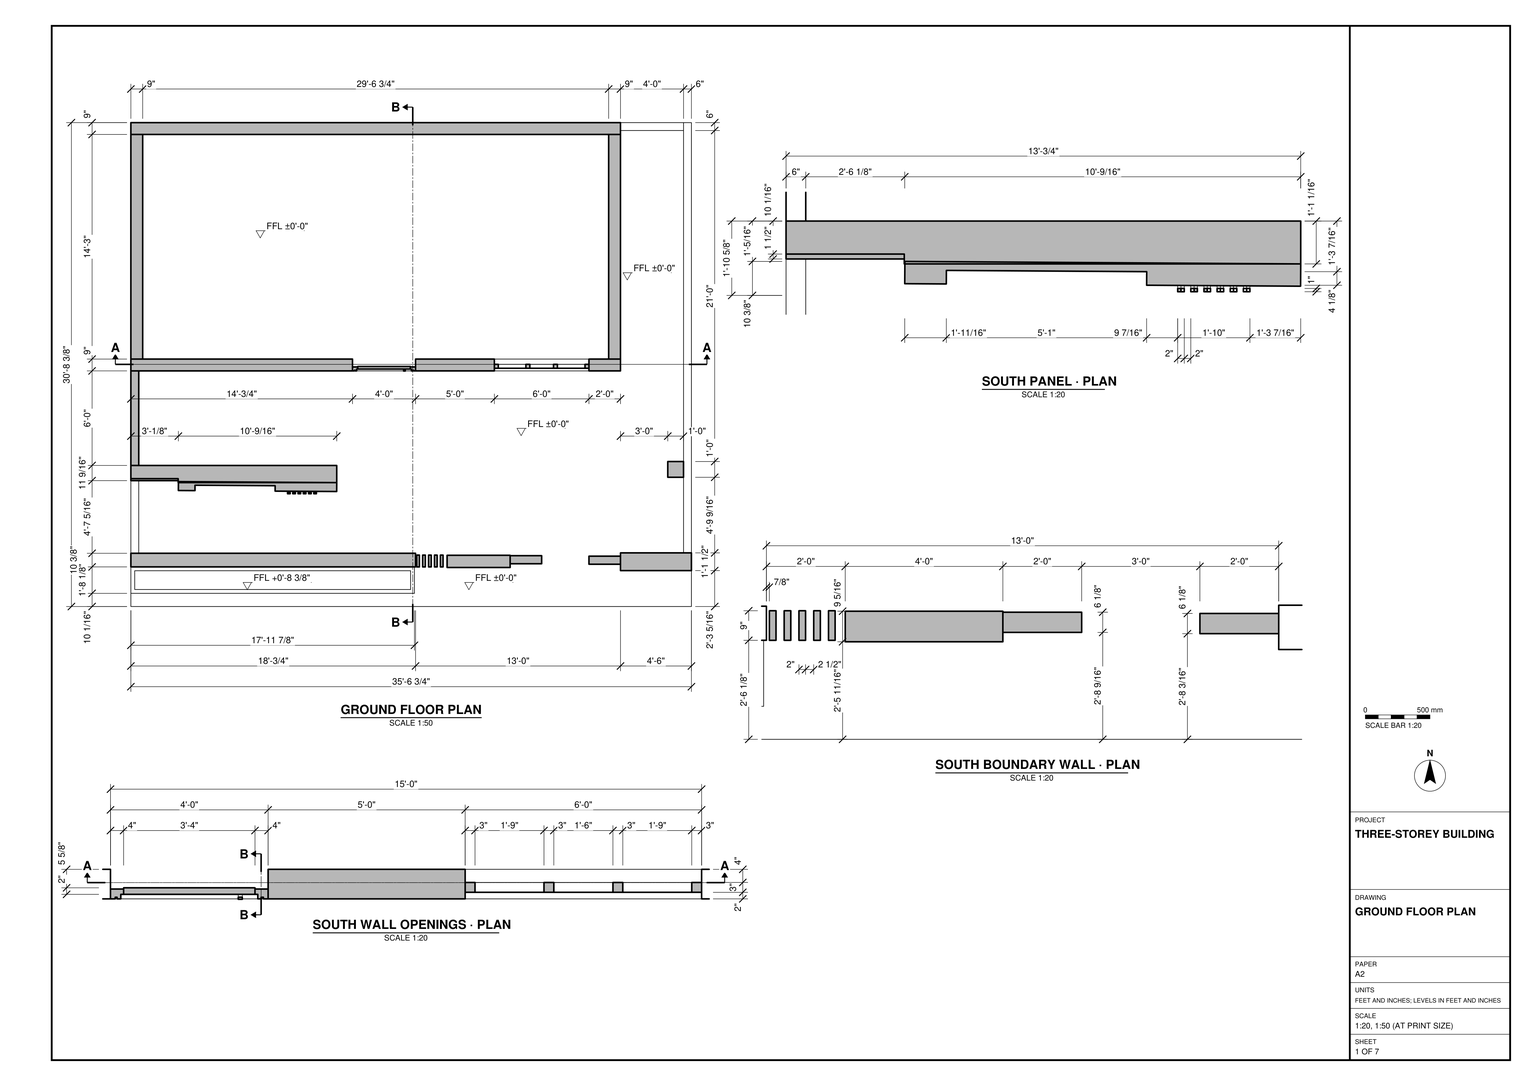
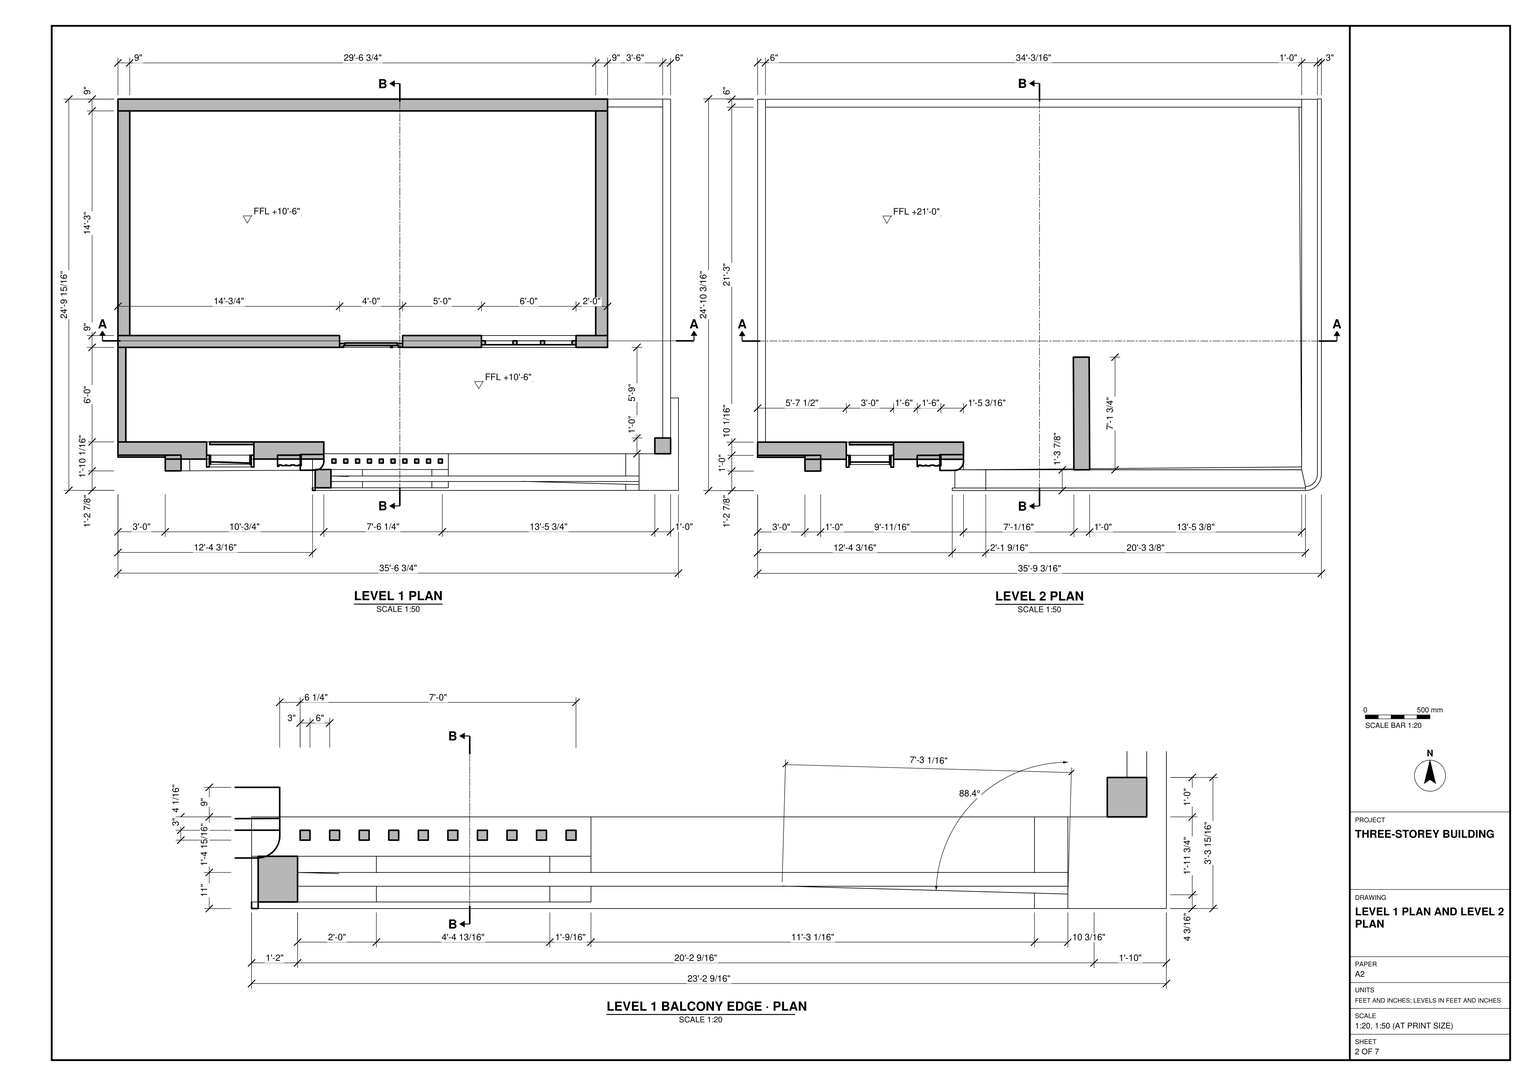
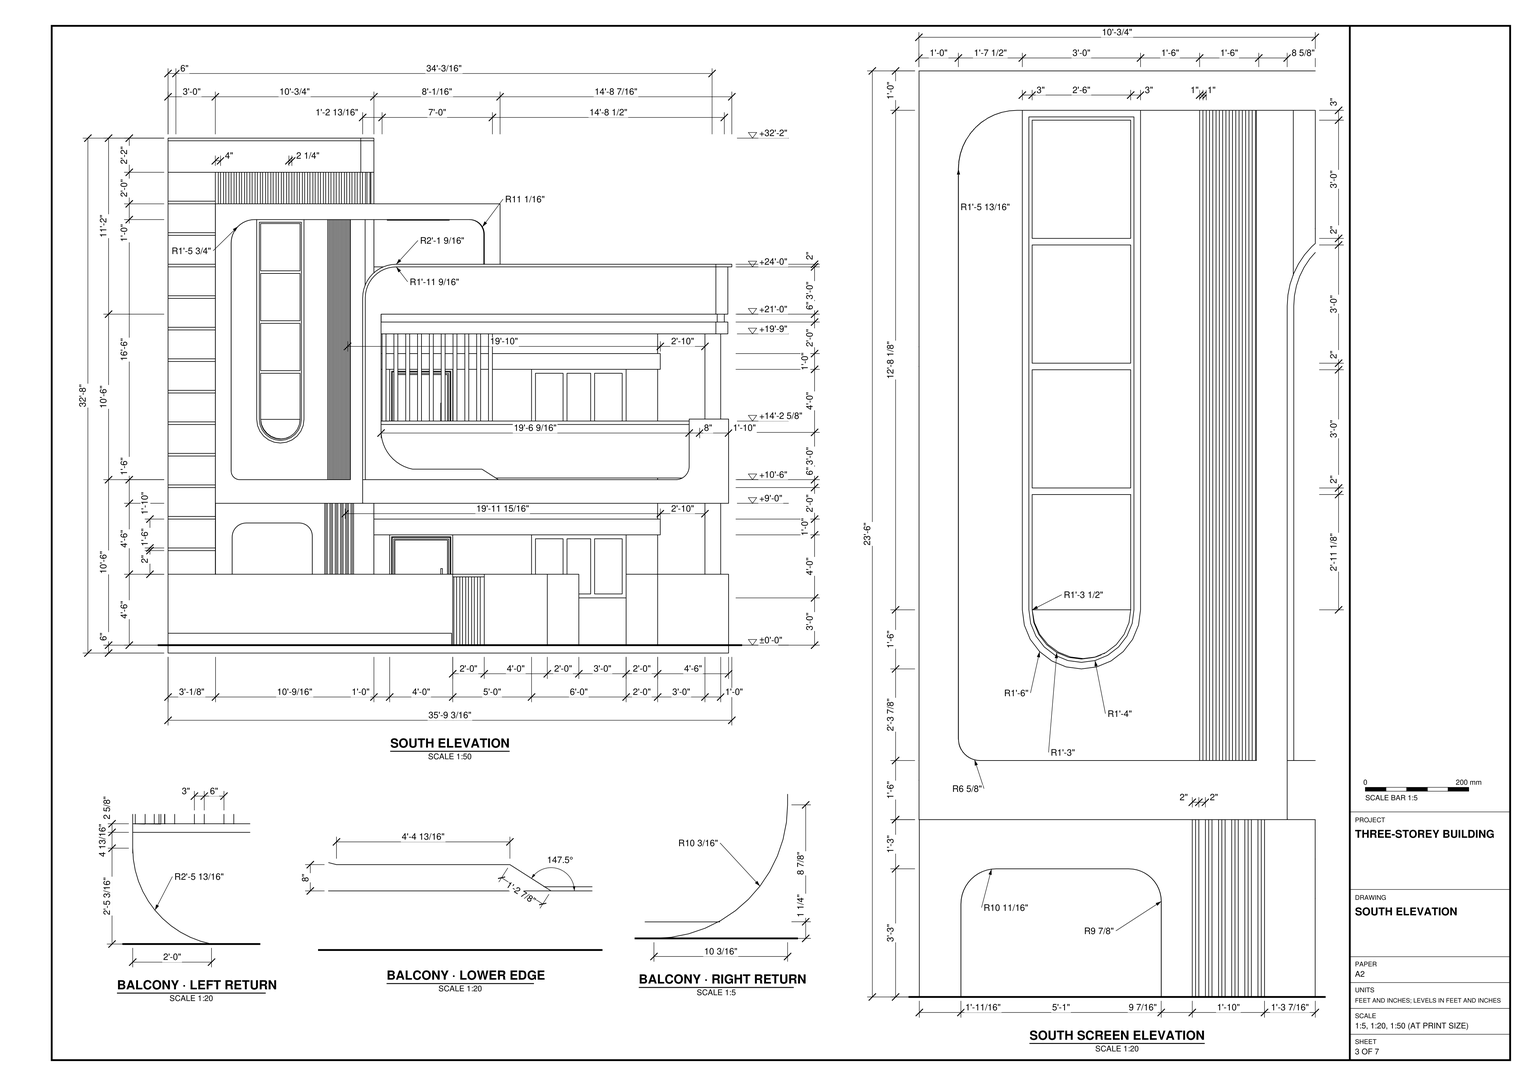
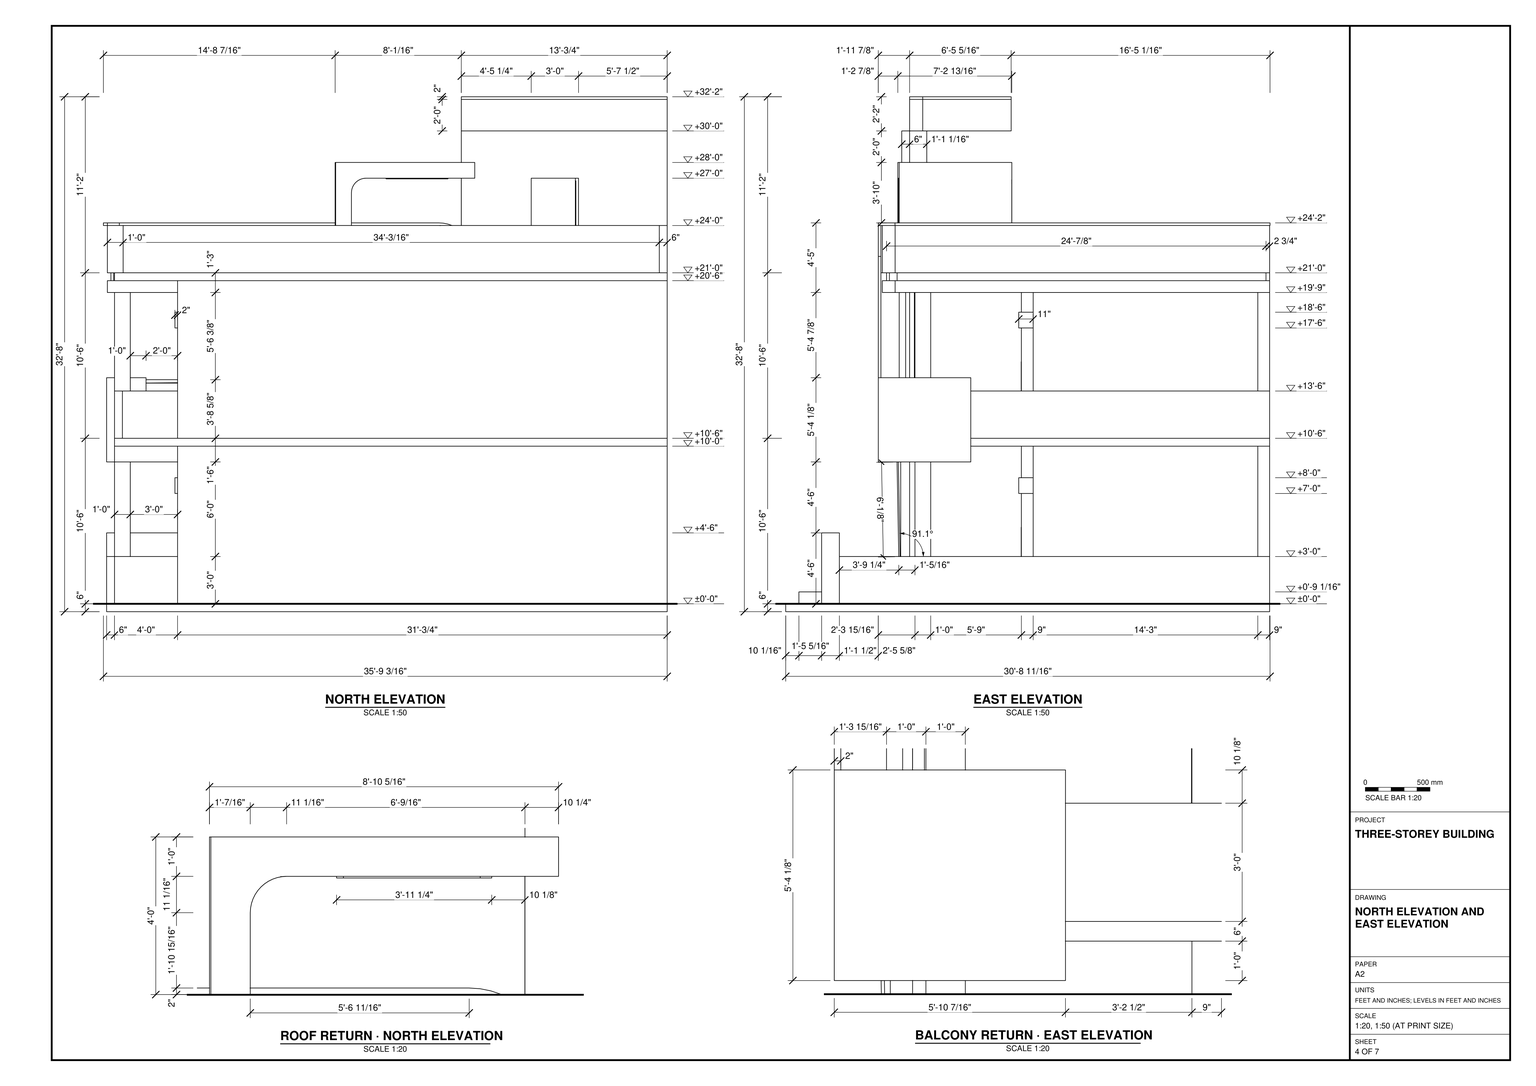
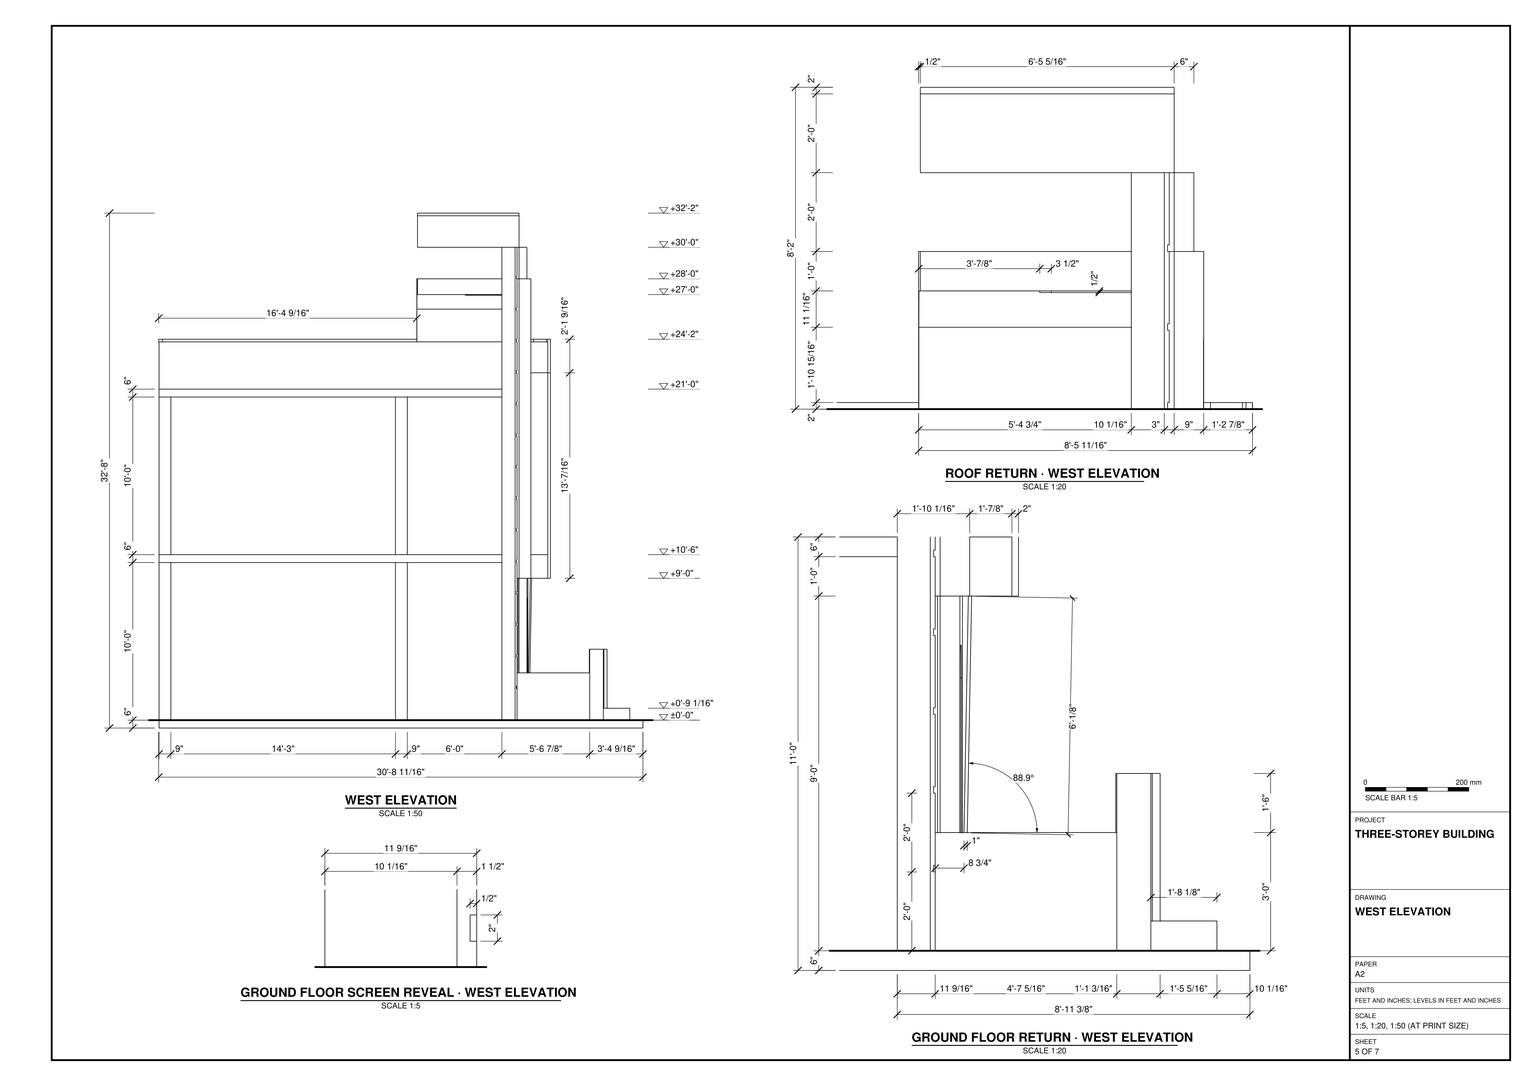
Build the three-storey building in SketchUp from task_files/diagram_01.pdf. Work in feet and inches. Set the overall east–west width to 35'-9 3/16", the north–south depth to 30'-8 11/16" and the total height to 32'-8". Use finished floor levels of ±0'-0", +10'-6" and +21'-0".

On the ground floor and Level 1, place the rectangular enclosure to the north. Model its 9" walls with a door opening and a wider, divided window opening facing south. Follow the plans for the thicknesses and offsets of the other walls, slabs, screens and parapets. Keep the ground-floor boundary wall distinct from the south screen behind it, leaving the entrance gap as drawn.

Project the Level 1 balcony in front of the enclosed space. Shape its curved returns and stepped lower edge, and place the vertical fins at its west end. Carry the tall south screen above the main flat roof, including its narrow round-bottomed inset, ribbed strip and slatted upper section. Follow the sheets for any stairs, built-in joinery and main furniture. Decor and loose items may be any suitable library components.

Keep shell elements and individual furniture or joinery pieces in separate groups or components, and use components for repeated parts. Save one SketchUp model as output_files/three_storey_building_with_a_screened_south_balcony.skp.

# SketchUp Ruby script. Lengths in inches.
U = 1.inch
M = Sketchup.active_model
def pt(a) = Geom::Point3d.new(a.map { |v| v * U })
def face(e, loops, mat)
  f = e.add_face(loops[0].map { |a| pt(a) })
  loops[1..].each { |l| e.add_face(l.map { |a| pt(a) }).erase! }
  f.material = f.back_material = mat if mat
  f
end
# faces: each face lists its corners as indices into pts; further lists are holes
def faces(e, pts, list, mat = nil) = list.each { |f| face(e, (f[0].is_a?(Array) ? f : [f]).map { |l| l.map { |i| pts[i] } }, mat) }
# xy, xz, yz: faces in a plane at the given z, y or x. An outline is a flat list of corners, or four numbers for a rectangle; further outlines are holes
def ring(l) = l.size == 4 ? [[l[0], l[1]], [l[2], l[1]], [l[2], l[3]], [l[0], l[3]]] : l.each_slice(2).to_a
def flat(e, list, mat, &to3) = list.each { |f| face(e, (f[0].is_a?(Array) ? f : [f]).map { |l| ring(l).map { |u, v| to3.(u, v) } }, mat) }
def xy(e, z, list, mat = nil) = flat(e, list, mat) { |x, y| [x, y, z] }
def xz(e, y, list, mat = nil) = flat(e, list, mat) { |x, z| [x, y, z] }
def yz(e, x, list, mat = nil) = flat(e, list, mat) { |y, z| [x, y, z] }
def lines(e, pts, list) = list.each { |a, b| e.add_line(pt(pts[a]), pt(pts[b])) }
# prism: a flat outline (further loops are holes) pulled along v
def prism(e, loops, v, mat = nil)
  f = face(e, loops, mat); d = Geom::Vector3d.new(v.map { |x| x * U })
  f.pushpull(f.normal.samedirection?(d) ? d.length : -d.length)
end
def box(e, o, s, mat = nil) = prism(e, [[o, [o[0] + s[0], o[1], o[2]], [o[0] + s[0], o[1] + s[1], o[2]], [o[0], o[1] + s[1], o[2]]]], [0, 0, s[2]], mat)
def at(x, y, z, deg = 0) = Geom::Transformation.translation(pt([x, y, z])) * Geom::Transformation.rotation(ORIGIN, Z_AXIS, deg.degrees)
def axes(o, x, y, z) = Geom::Transformation.new([*x, 0, *y, 0, *z, 0, *pt(o).to_a, 1])
def part(name) = M.definitions.add(name)
# library, detail: a bought-in or finely detailed component or shape, given as its bounding box
def library(name, o, s) = part(name).tap { |d| box(d.entities, o, s) }
def detail(e, o, s) = box(e.add_group.entities, o, s)
def put(e, d, t, mat = nil) = e.add_instance(d, t).tap { |i| i.material = mat if mat }
def group(e, t, mat = nil) = e.add_group.tap { |g| g.transformation = t; g.material = mat if mat }.entities
root = M.entities
M.materials.add("[Aluminum]").color = [179, 179, 179]
M.materials.add("[Color M00]").color = [255, 255, 255]
M.materials.add("[Color M04]").color = [142, 142, 142]
M.materials.add("[Color M06]").color = [86, 86, 86]
M.materials.add("[Color M09]").color = [0, 0, 0]
M.materials.add("[Field Rectangle Tile]").color = [242, 233, 221]
M.materials.add("[Grass Dark Green]").color = [106, 157, 55]
M.materials.add("[Metal Rusted]").color = [184, 117, 91]
M.materials.add("[Translucent Glass Gray]").color = [128, 128, 128]
M.materials.add("[Wood Bamboo]").color = [177, 105, 43]
M.materials.add("[Wood Board Cork]").color = [181, 169, 96]
M.materials.add("[Wood Cherry Original]").color = [152, 86, 42]
M.materials.add("[Wood Fence with Lattice]").color = [109, 68, 39]
M.materials.add("[Wood Floor]").color = [112, 76, 44]
M.materials.add("[Wood Veneer 01]").color = [120, 70, 37]
c1 = part("Group\#3")
prism(c1.entities,[[[0,3,0],[0,3,48],[72,3,48],[72,3,0]],[[24,3,3],[24,3,45],[3,3,45],[3,3,3]],[[69,3,45],[48,3,45],[48,3,3],[69,3,3]],[[45,3,3],[45,3,45],[27,3,45],[27,3,3]]],[0,-3,0])
c2 = part("Group\#4")
xz(c2.entities,0,[[0,0,21,42]])
c3 = part("Group\#5")
xz(c3.entities,0,[[0,0,18,42]])
c4 = part("Group\#6")
xz(c4.entities,0,[[0,0,21,42]])
c5 = part("Group\#7")
xy(c5.entities,0,[[0,0,48,3]])
xy(c5.entities,1.44,[[1.44,0,46.56,0.5]])
xy(c5.entities,2,[[2,0,46,0.5]])
xy(c5.entities,3.15,[[3.15,0,44.85,1.375]])
xy(c5.entities,4,[[4,1.375,44,3]])
xy(c5.entities,80,[[4,1.375,44,3]])
xy(c5.entities,80.85,[[3.15,0,44.85,1.375]])
xy(c5.entities,82,[[2,0,46,0.5]])
xy(c5.entities,82.56,[[1.44,0,46.56,0.5]])
xy(c5.entities,84,[[0,0,48,3]])
xz(c5.entities,0,[[[0,0,48,84],[1.44,1.44,46.56,82.56]],[[2,2,46,82],[3.15,3.15,44.85,80.85]]])
xz(c5.entities,0.5,[[[1.44,1.44,46.56,82.56],[2,2,46,82]]])
xz(c5.entities,1.375,[[[3.15,3.15,44.85,80.85],[4,4,44,80]]])
xz(c5.entities,3,[[[0,0,48,84],[4,4,44,80]]])
yz(c5.entities,0,[[0,0,3,84]])
yz(c5.entities,1.44,[[0,1.44,0.5,82.56]])
yz(c5.entities,2,[[0,2,0.5,82]])
yz(c5.entities,3.15,[[0,3.15,1.375,80.85]])
yz(c5.entities,4,[[1.375,4,3,80]])
yz(c5.entities,44,[[1.375,4,3,80]])
yz(c5.entities,44.85,[[0,3.15,1.375,80.85]])
yz(c5.entities,46,[[0,2,0.5,82]])
yz(c5.entities,46.56,[[0,1.44,0.5,82.56]])
yz(c5.entities,48,[[0,0,3,84]])
c6 = part("Group\#8")
box(c6.entities,[0,-2,0],[40,2,76])
c7 = part("Group\#13")
prism(c7.entities,[[[1.25,1.5,24.92],[1.25,1.5,26.5625],[1.25,0,26.5625],[1.25,0,0],[1.25,1.5,0],[1.25,1.5,1.64],[1.25,0.64,1.64],[1.25,0.64,24.92]]],[-1.25,0,0])
c8 = part("Group\#12")
box(c8.entities,[0,0,0],[9,171,120])
c9 = library("Group\#19",[-2,-2.87,-18],[281.03,278.7,182])
c10 = part("Group\#33")
box(c10.entities,[0,0,0],[2.28,6,24])
c11 = part("Group\#60")
prism(c11.entities,[[[0,3,0.02],[1,3,0.02],[1,2,0],[0,2,0]]],[0.01,-2,107.98])
c12 = part("Group\#37")
box(c12.entities,[0,0,0],[3,3,120])
xy(root,132,[[150.78,85.84,150.98,85.85,151.19,85.87,151.39,85.91,151.6,85.96,151.79,86.02,151.99,86.09,152.17,86.18,152.36,86.28,152.53,86.39,150.16,85.9,150.36,85.86]])
xy(root,366,[[0,94.33,0,171.62,156.72,171.62,156.72,104.31,156.64,103.01,156.38,101.73,155.96,100.49,155.39,99.32,154.66,98.24,153.8,97.26,152.82,96.39,151.73,95.67,150.5625,95.09,149.33,94.67,148.05,94.42,146.75,94.33]])
xy(root,390,[[0,94.33,146.75,94.33,148.05,94.42,149.33,94.67,150.5625,95.09,151.73,95.67,152.82,96.39,153.8,97.26,154.66,98.24,155.39,99.32,155.96,100.49,156.38,101.73,156.64,103.01,156.72,104.31,156.72,171.62,0,171.62]])
xy(root,392,[[0,94.33,146.75,94.33,148.05,94.42,149.33,94.67,150.5625,95.09,151.73,95.67,152.82,96.39,153.8,97.26,154.66,98.24,155.39,99.32,155.96,100.49,156.38,101.73,156.64,103.01,156.72,104.31,156.72,171.62,0,171.62]])
xz(root,85.88,[[148.16,114,150.16,132,148.16,132]])
xz(root,94.33,[[0,366,146.75,390]])
xz(root,94.33,[[0,390,146.75,392]],"[Color M09]")
xz(root,171.62,[[0,366,156.72,390],[0,390,156.72,392]])
yz(root,0,[[94.33,366,171.62,390],[94.33,390,171.62,392]])
yz(root,156.72,[[104.31,366,171.62,390]])
yz(root,156.72,[[104.31,390,171.62,392]],"[Color M09]")
# 27 loose lines left out
p = [[148.05,94.42,390],[146.75,94.33,390],[146.75,94.33,366],[148.05,94.42,366],[149.33,94.67,390],[149.33,94.67,366],
  [150.5625,95.09,390],[150.5625,95.09,366],[151.73,95.67,390],[151.73,95.67,366],[152.82,96.39,390],[152.82,96.39,366],
  [153.8,97.26,390],[153.8,97.26,366],[154.66,98.24,390],[154.66,98.24,366],[155.39,99.32,390],[155.39,99.32,366],
  [155.96,100.49,390],[155.96,100.49,366],[156.38,101.73,390],[156.38,101.73,366],[156.64,103.01,390],[156.64,103.01,366],
  [156.72,104.31,390],[156.72,104.31,366],[148.05,94.42,392],[146.75,94.33,392],[149.33,94.67,392],[150.5625,95.09,392],
  [151.73,95.67,392],[152.82,96.39,392],[153.8,97.26,392],[154.66,98.24,392],[155.39,99.32,392],[155.96,100.49,392],
  [156.38,101.73,392],[156.64,103.01,392],[156.72,104.31,392]]
faces(root,p,[[0,1,2,3],[4,0,3,5],[6,4,5,7],[8,6,7,9],[10,8,9,11],[12,10,11,13],[14,12,13,15],[16,14,15,17],
  [18,16,17,19],[20,18,19,21],[22,20,21,23],[24,22,23,25]])
faces(root,p,[[1,0,26,27],[0,4,28,26],[4,6,29,28],[6,8,30,29],[8,10,31,30],[10,12,32,31],[12,14,33,32],[14,16,34,33],
  [16,18,35,34],[18,20,36,35],[20,22,37,36],[22,24,38,37]],"[Color M09]")
g1 = group(root,at(-107.28,-0.61,0))
xy(g1,0,[[107.28,0.61,534,369]])
xy(g1,6,[[107.28,0.61,534,369]],"[Field Rectangle Tile]")
xz(g1,0.61,[[107.28,0,534,6]])
xz(g1,369,[[107.28,0,534,6]])
yz(g1,107.28,[[0.61,0,369,6]])
yz(g1,534,[[0.61,0,369,6]])
g2 = group(root,at(-107.28,179.39,6))
prism(g2,[[[480,9,0],[324,9,0],[324,9,84],[276,9,84],[276,9,0],[107.28,9,0],[107.28,9,120],[480,9,120]],[[384,9,84],[384,9,36],[456,9,36],[456,9,84]]],[0,-9,0])
put(root,c1,at(276.72,181.39,42),"[Color M09]")
put(root,c2,at(324.72,181.39,45),"[Translucent Glass Gray]")
put(root,c3,at(303.72,181.39,45),"[Translucent Glass Gray]")
put(root,c4,at(279.72,181.39,45),"[Translucent Glass Gray]")
put(root,c5,at(168.72,179.39,6),"[Wood Veneer 01]")
put(root,c6,at(172.72,182.76,10),"[Wood Cherry Original]")
g3 = group(root,at(156.72,177.39,90),"[Wood Board Cork]")
prism(g3,[[[-21.9375,2,0],[216,2,0],[216,11,0],[218,11,0],[218,0,0],[-21.9375,0,0]]],[0,0,12])
g4 = group(root,at(-107.28,359.39,6))
box(g4,[107.28,0,0],[372.72,9,120])
g5 = group(root,at(363.72,188.39,6))
box(g5,[0,0,0],[9,171,120])
put(root,c7,at(207.62,179.26,37.75),"[Aluminum]")
put(root,c8,at(0,188.39,6))
g6 = group(root,at(-17.28,179.39,126))
prism(g6,[[[174,-72,0],[17.28,-72,0],[17.28,189,0],[438,189,0],[438,-81,0],[174,-81,0]]],[0,0,6])
put(root,c4,at(279.72,181.39,171),"[Translucent Glass Gray]")
put(root,c6,at(172.72,182.76,136),"[Wood Cherry Original]")
put(root,c3,at(303.72,181.39,171),"[Translucent Glass Gray]")
put(root,c2,at(324.72,181.39,171),"[Translucent Glass Gray]")
put(root,c5,at(168.72,179.39,132),"[Wood Veneer 01]")
g7 = group(root,at(156.72,177.39,216),"[Wood Board Cork]")
prism(g7,[[[-20,2,0],[216,2,0],[216,11,0],[218,11,0],[218,0,0],[-20,0,0]]],[0,0,12])
put(root,c7,at(207.62,179.26,163.75),"[Aluminum]")
put(root,c8,at(0,188.39,132))
g8 = group(root,at(-107.28,179.39,132))
prism(g8,[[[480,9,0],[324,9,0],[324,9,84],[276,9,84],[276,9,0],[107.28,9,0],[107.28,9,120],[480,9,120]],[[384,9,84],[384,9,36],[456,9,36],[456,9,84]]],[0,-9,0])
g9 = group(root,at(-107.28,359.39,132))
box(g9,[107.28,0,0],[372.72,9,120])
g10 = group(root,at(363.72,188.39,132))
box(g10,[0,0,0],[9,171,120])
g11 = group(root,at(-17.28,179.39,252))
prism(g11,[[[174,-72,0],[17.28,-72,0],[17.28,189,0],[438,189,0],[438,-93.06,0],[174,-93.06,0]]],[0,0,6])
put(root,c1,at(276.72,181.39,168),"[Color M09]")
put(root,c9,axes([150.16,73.55,132],[1,0,0],[0,1.07,0],[0,0,1]),"[Color M00]")
g12 = group(root,at(162.16,76.76,252),"[Wood Board Cork]")
prism(g12,[[[259.21,288.86,0],[261.29,8.04,0],[261.25,7.28,0],[261.12,6.53,0],[260.89,5.81,0],[260.58,5.12,0],[260.19,4.49,0],[259.73,3.91,0],[259.2,3.4,0],[258.61,2.98,0],[257.97,2.63,0],[257.3,2.38,0],[256.6,2.23,0],[255.89,2.17,0],[0.07,0,0],[0,9.63,0],[252,11.77,0],[249.95,288.78,0]]],[0,0,6])
g13 = group(root,at(408.72,98.39,132))
xy(g13,0,[[0,0,12,12]])
xy(g13,122.1875,[[0,0,12,12]])
xz(g13,0,[[0,0,12,111],[0,111,12,122.1875]])
xz(g13,12,[[0,0,12,122.1875]])
yz(g13,0,[[0,0,12,122.1875]])
yz(g13,12,[[0,0,12,111],[0,111,12,122.1875]])
g14 = group(root,at(408.72,98.39,-8.1875))
box(g14,[0,0,14.1875],[12,12,108])
g15 = group(root,at(121.5,89.33,132),"[Wood Veneer 01]")
xy(g15,0,[[0,-0.5,0,8,18,8,18,0,17,0,17,0.5,16,0.5,16,0,13,0,13,0.5,10,0.5,10,0,7,0,7,0.5,6,0.5,6,0,3,0,3,0.5,1,0.5,1,-0.5],[16,0.375,17,0.5]])
xy(g15,198,[[0,-0.5,1,-0.5,1,0.5,3,0.5,3,0,6,0,6,0.5,7,0.5,7,0,10,0,10,0.5,13,0.5,13,0,16,0,16,0.5,17,0.5,17,0,18,0,18,8,0,8],[16,0.375,17,0.5],[16,0.375,17,0.5]])
xz(g15,-0.5,[[0,0,1,198]])
xz(g15,0,[[3,0,4,198],[4,0,5,198],[5,0,6,198],[7,0,8,198],[8,0,9,198],
  [9,0,10,198],[13,0,14,198],[14,0,15,198],[15,0,16,198],[17,0,18,198]])
xz(g15,0.375,[[16,0,17,198]])
xz(g15,0.5,[[1,0,2,198],[2,0,3,198],[6,0,7,198],[10,0,11,198],[11,0,12,198],
  [12,0,13,198],[16,0,17,198]])
xz(g15,8,[[0,0,18,198]])
yz(g15,0,[[-0.5,0,8,198]])
yz(g15,1,[[-0.5,0,0.5,198]])
yz(g15,3,[[0,0,0.5,198]])
yz(g15,6,[[0,0,0.5,198]])
yz(g15,7,[[0,0,0.5,198]])
yz(g15,10,[[0,0,0.5,198]])
yz(g15,13,[[0,0,0.5,198]])
yz(g15,16,[[0,0,0.375,198],[0.375,0,0.5,198]])
yz(g15,17,[[0,0,0.375,198],[0.375,0,0.5,198]])
yz(g15,18,[[0,0,8,198]])
g16 = group(root,at(36,85.33,114))
prism(g16,[[[178.08,47.84,215.5],[178.08,18.1,215.5],[178.05,17.71,215.5],[177.98,17.32,215.5],[177.85,16.95,215.5],[177.68,16.6,215.5],[177.46,16.28,215.5],[177.2,15.98,215.5],[176.91,15.72,215.5],[176.58,15.51,215.5],[176.23,15.33,215.5],[175.86,15.21,215.5],[175.48,15.13,215.5],[175.09,15.11,215.5],[133.63,15.11,215.5],[133.26,15.13,215.5],[132.91,15.2,215.5],[132.56,15.32,215.5],[132.23,15.48,215.5],[131.92,15.68,215.5],[131.65,15.93,215.5],[131.41,16.2,215.5],[131.2,16.51,215.5],[131.04,16.84,215.5],[130.92,17.18,215.5],[130.85,17.54,215.5],[130.83,17.91,215.5],[130.83,46.4,215.5],[130.86,46.86,215.5],[130.95,47.3125,215.5],[131.1,47.75,215.5],[131.3,48.16,215.5],[131.56,48.54,215.5],[131.86,48.89,215.5],[132.2,49.19,215.5],[132.59,49.45,215.5],[133,49.65,215.5],[133.43,49.8,215.5],[133.88,49.89,215.5],[134.34,49.92,215.5],[176,49.92,215.5],[176.27,49.9,215.5],[176.54,49.85,215.5],[176.79,49.76,215.5],[177.04,49.64,215.5],[177.26,49.49,215.5],[177.47,49.31,215.5],[177.65,49.1,215.5],[177.8,48.88,215.5],[177.92,48.63,215.5],[178.01,48.375,215.5],[178.0625,48.11,215.5]]],[0,0,0.5],"[Wood Cherry Original]")
xy(g16,0,[[0.06,0,0,12,120.72,12.59,120.75,7.34,120.75,7.33,120.7,6.46,120.53,5.59,120.25,4.75,119.86,3.96,119.375,3.22,118.8,2.56,118.13,1.97,117.4,1.48,116.61,1.08,115.78,0.79,114.91,0.62,114.03,0.55]])
xy(g16,18,[[18.67,0.09,102.78,0.5,102.72,12.5,18.62,12.09]])
xy(g16,144,[[204.78,1,204.36,86.74,216.36,86.8,216.78,1.05]])
xy(g16,216,[[29.88,0.14,29.82,12.14,102.72,12.5,102.78,0.5],[102.78,0.5,102.72,12.5,110.85,12.54,110.49,86.29,193.29,86.69,193.71,0.94,114.02,0.55],[102.78,0.5,114.02,0.55,114.91,0.62,115.77,0.79,116.61,1.08,117.4,1.48,118.13,1.97,118.79,2.56,119.37,3.22,119.86,3.96,120.24,4.75,120.52,5.59,120.69,6.46,120.74,7.34,120.72,12.59,110.85,12.54,102.72,12.5]])
xy(g16,228,[[0.06,0,216.78,1.05,216.36,86.8,110.49,86.29,110.85,12.54,0,12]])
# 1 loose lines left out
p = [[0,12,228],[0,12,0],[0.06,0,0],[0.06,0,228],[114.03,0.55,0],[114.02,0.55,216],
  [193.71,0.94,216],[195.16,0.95,215.91],[196.58,0.96,215.62],[197.95,0.96,215.16],[199.25,0.97,214.52],[200.45,0.97,213.71],
  [201.54,0.98,212.76],[202.49,0.98,211.67],[203.3,0.99,210.47],[203.9375,0.99,209.17],[204.4,0.99,207.8],[204.69,0.99,206.375],
  [204.78,1,204.93],[204.78,1,144],[216.78,1.05,144],[216.78,1.05,228],[102.78,0.5,18],[18.67,0.09,18],
  [17.8125,0.09,18.06],[16.96,0.08,18.23],[16.14,0.08,18.5],[15.37,0.07,18.89],[14.65,0.07,19.37],[14,0.07,19.9375],
  [13.43,0.06,20.59],[12.94,0.0625,21.31],[12.5625,0.0625,22.09],[12.28,0.06,22.9],[12.11,0.06,23.75],[12.06,0.06,24.62],
  [12.06,0.06,198.18],[12.21,0.06,200.5],[12.67,0.0625,202.79],[13.41,0.06,205],[14.45,0.07,207.09],[15.74,0.08,209.03],
  [17.28,0.08,210.78],[19.03,0.09,212.32],[20.97,0.1,213.61],[23.06,0.11,214.64],[25.27,0.12,215.39],[27.55,0.13,215.85],
  [29.88,0.14,216],[102.78,0.5,216],[114.91,0.62,0],[114.91,0.62,216],[115.78,0.79,0],[115.77,0.79,216],
  [116.61,1.08,0],[116.61,1.08,216],[117.4,1.48,0],[117.4,1.48,216],[118.13,1.97,0],[118.13,1.97,216],
  [118.8,2.56,0],[118.79,2.56,216],[119.375,3.22,0],[119.37,3.22,216],[119.86,3.96,0],[119.86,3.96,216],
  [120.25,4.75,0],[120.24,4.75,216],[120.53,5.59,0],[120.52,5.59,216],[120.7,6.46,0],[120.69,6.46,216],
  [120.75,7.34,0],[120.74,7.34,216],[120.75,7.33,0],[120.72,12.59,0],[120.72,12.59,216],[110.85,12.54,228],
  [110.85,12.54,216],[102.72,12.5,18],[102.72,12.5,216],[29.82,12.14,216],[27.5,12.13,215.85],[25.21,12.12,215.39],
  [23,12.11,214.64],[20.91,12.1,213.61],[18.97,12.09,212.32],[17.22,12.08,210.78],[15.68,12.08,209.03],[14.39,12.07,207.09],
  [13.36,12.06,205],[12.61,12.0625,202.79],[12.15,12.06,200.5],[12,12.06,198.18],[12,12.06,24.62],[12,12.06,18],
  [18.62,12.09,18],[17.75,12.09,18.06],[12.06,12.06,23.75],[12.23,12.06,22.9],[12.5,12.0625,22.09],[12.89,12.0625,21.31],
  [13.37,12.06,20.59],[13.9375,12.07,19.9375],[14.59,12.07,19.37],[15.31,12.07,18.89],[16.08,12.08,18.5],[16.9,12.08,18.23],
  [204.36,86.74,204.93],[204.36,86.74,144],[216.36,86.8,144],[216.36,86.8,228],[193.29,86.69,216],[110.49,86.29,216],
  [110.49,86.29,228],[204.27,86.74,206.375],[203.99,86.74,207.8],[203.52,86.74,209.17],[202.88,86.74,210.47],[202.08,86.73,211.67],
  [201.12,86.73,212.76],[200.03,86.72,213.71],[198.83,86.72,214.52],[197.53,86.71,215.16],[196.16,86.7,215.62],[194.74,86.7,215.91]]
faces(g16,p,[[0,1,2,3],[[4,5,6,7,8,9,10,11,12,13,14,15,16,17,18,19,20,21,3,2],[22,23,24,25,26,27,28,29,30,31,32,33,34,35,36,37,38,39,40,41,42,43,44,45,46,47,48,49]],[50,51,5,4],[52,53,51,50],[54,55,53,52],[56,57,55,54],[58,59,57,56],[60,61,59,58],
  [62,63,61,60],[64,65,63,62],[66,67,65,64],[68,69,67,66],[70,71,69,68],[72,73,71,70,74],[73,72,75,76],[[0,77,78,76,75,1],[79,80,81,82,83,84,85,86,87,88,89,90,91,92,93,94,95,96]],
  [24,23,96,97],[79,22,49,80],[97,96,95,94,98,99,100,101,102,103,104,105,106,107],[25,24,97,107],[26,25,107,106],[27,26,106,105],[28,27,105,104],[29,28,104,103],
  [30,29,103,102],[31,30,102,101],[32,31,101,100],[33,32,100,99],[34,33,99,98],[35,34,98,94],[36,35,94,93],[18,108,109,19],
  [20,110,111,21],[112,113,114,111,110,109,108,115,116,117,118,119,120,121,122,123,124,125],[93,92,37,36],[92,91,38,37],[91,90,39,38],[17,115,108,18],[90,89,40,39],[16,116,115,17],
  [89,88,41,40],[15,117,116,16],[88,87,42,41],[14,118,117,15],[13,119,118,14],[87,86,43,42],[12,120,119,13],[86,85,44,43],
  [11,121,120,12],[85,84,45,44],[10,122,121,11],[9,123,122,10],[84,83,46,45],[8,124,123,9],[83,82,47,46],[7,125,124,8],
  [82,81,48,47],[6,112,125,7],[78,77,114,113]])
g17 = group(root,at(-17.28,98.39,6))
xy(g17,0,[[53.28,-4.05,53.28,-1.05,17.28,-1.05,17.28,9,174,9,174,-4.05]])
xy(g17,324,[[84.78,-4.05,120.78,9]])
xy(g17,360,[[53.28,-4.05,174,-4.05,174,9,17.28,9,17.28,-1.05,53.28,-1.05]])
xz(g17,-4.05,[[[53.28,0,174,360],[102.78,153.9,98.12,154.51,93.78,156.31,90.05,159.17,87.19,162.9,85.39,167.24,84.78,171.9,84.78,324,120.78,324,120.78,171.9,120.17,167.24,118.37,162.9,115.51,159.17,111.78,156.31,107.4375,154.51]]])
xz(g17,-1.05,[[17.28,0,53.28,360]])
xz(g17,9,[[[17.28,0,174,360],[102.78,153.9,107.4375,154.51,111.78,156.31,115.51,159.17,118.37,162.9,120.17,167.24,120.78,171.9,120.78,324,84.78,324,84.78,171.9,85.39,167.24,87.19,162.9,90.05,159.17,93.78,156.31,98.12,154.51]]])
yz(g17,17.28,[[-1.05,0,9,360]])
yz(g17,53.28,[[-4.05,0,-1.05,360]])
yz(g17,84.78,[[-4.05,171.9,9,324]])
yz(g17,120.78,[[-4.05,171.9,9,324]])
yz(g17,174,[[-4.05,0,9,360]])
# 1 loose lines left out
p = [[98.12,9,154.51],[98.12,-4.05,154.51],[102.78,-4.05,153.9],[102.78,9,153.9],[107.4375,-4.05,154.51],[107.4375,9,154.51],
  [93.78,9,156.31],[93.78,-4.05,156.31],[111.78,-4.05,156.31],[111.78,9,156.31],[90.05,9,159.17],[90.05,-4.05,159.17],
  [115.51,-4.05,159.17],[115.51,9,159.17],[87.19,9,162.9],[87.19,-4.05,162.9],[118.37,-4.05,162.9],[118.37,9,162.9],
  [85.39,9,167.24],[85.39,-4.05,167.24],[120.17,-4.05,167.24],[120.17,9,167.24],[84.78,9,171.9],[84.78,-4.05,171.9],
  [120.78,-4.05,171.9],[120.78,9,171.9]]
faces(g17,p,[[0,1,2,3],[3,2,4,5],[6,7,1,0],[5,4,8,9],[10,11,7,6],[9,8,12,13],[14,15,11,10],[13,12,16,17],
  [18,19,15,14],[17,16,20,21],[22,23,19,18],[21,20,24,25]])
g18 = group(root,at(67.5,97.33,159.9),"[Color M06]")
xy(g18,53.1,[[3,-7,33,0]])
xy(g18,55.1,[[3,-7,33,0]],"[Color M00]")
xy(g18,91.1,[[3,-7,33,0]])
xy(g18,93.1,[[3,-7,33,0]])
xy(g18,129.1,[[3,-7,33,0]])
xy(g18,131.1,[[3,-7,33,0]])
xy(g18,167.1,[[3,-7,33,0]])
xy(g18,168.1,[[2,-9,34,-7],[2,-7,34,0]])
xy(g18,170.1,[[0,-9,36,0]])
xz(g18,-9,[[[18,0,22.66,0.61,27,2.41,30.73,5.27,33.59,9,35.39,13.34,36,18,36,170.1,0,170.1,0,18,0.61,13.34,2.41,9,5.27,5.27,9,2.41,13.34,0.61],[18,2,13.86,2.55,10,4.14,6.6875,6.6875,4.14,10,2.55,13.86,2,18,2,168.1,34,168.1,34,18,33.45,13.86,31.86,10,29.3125,6.6875,26,4.14,22.14,2.55]]])
xz(g18,-7,[[[18,2,13.86,2.55,10,4.14,6.6875,6.6875,4.14,10,2.55,13.86,2,18,2,168.1,34,168.1,34,18,33.45,13.86,31.86,10,29.3125,6.6875,26,4.14,22.14,2.55],[18,3,21.88,3.51,25.5,5.01,28.61,7.39,30.99,10.5,32.49,14.12,33,18,33,53.1,3,53.1,3,18,3.51,14.12,5.01,10.5,7.39,7.39,10.5,5.01,14.12,3.51],[3,55.1,33,91.1],[3,131.1,33,167.1],[3,93.1,33,129.1]]],"[Color M09]")
xz(g18,0,[[[18,0,13.34,0.61,9,2.41,5.27,5.27,2.41,9,0.61,13.34,0,18,0,170.1,36,170.1,36,18,35.39,13.34,33.59,9,30.73,5.27,27,2.41,22.66,0.61],[18,2,22.14,2.55,26,4.14,29.3125,6.6875,31.86,10,33.45,13.86,34,18,34,168.1,2,168.1,2,18,2.55,13.86,4.14,10,6.6875,6.6875,10,4.14,13.86,2.55]]])
yz(g18,0,[[-9,18,0,170.1]])
yz(g18,2,[[-9,18,-7,168.1],[-7,18,0,168.1]])
yz(g18,3,[[-7,18,0,53.1],[-7,55.1,0,91.1],[-7,93.1,0,129.1],[-7,131.1,0,167.1]])
yz(g18,33,[[-7,93.1,0,129.1],[-7,131.1,0,167.1]])
yz(g18,33,[[-7,18,0,53.1],[-7,55.1,0,91.1]],"[Color M00]")
yz(g18,34,[[-9,18,-7,168.1],[-7,18,0,168.1]])
yz(g18,36,[[-9,18,0,170.1]])
p = [[13.34,0,0.61],[18,0,0],[18,-9,0],[13.34,-9,0.61],[22.66,0,0.61],[22.66,-9,0.61],
  [9,0,2.41],[9,-9,2.41],[27,0,2.41],[27,-9,2.41],[18,-9,2],[18,-7,2],
  [13.86,-7,2.55],[13.86,-9,2.55],[22.14,-9,2.55],[22.14,-7,2.55],[18,0,2],[13.86,0,2.55],
  [22.14,0,2.55],[5.27,0,5.27],[5.27,-9,5.27],[30.73,0,5.27],[30.73,-9,5.27],[10,-7,4.14],
  [10,-9,4.14],[26,-9,4.14],[26,-7,4.14],[10,0,4.14],[26,0,4.14],[14.12,0,3.51],
  [18,0,3],[18,-7,3],[14.12,-7,3.51],[21.88,0,3.51],[21.88,-7,3.51],[10.5,0,5.01],
  [10.5,-7,5.01],[25.5,0,5.01],[25.5,-7,5.01],[6.6875,-7,6.6875],[6.6875,-9,6.6875],[29.3125,-9,6.6875],
  [29.3125,-7,6.6875],[6.6875,0,6.6875],[29.3125,0,6.6875],[7.39,0,7.39],[7.39,-7,7.39],[28.61,0,7.39],
  [28.61,-7,7.39],[2.41,0,9],[2.41,-9,9],[33.59,0,9],[33.59,-9,9],[4.14,-7,10],
  [4.14,-9,10],[31.86,-9,10],[31.86,-7,10],[4.14,0,10],[31.86,0,10],[5.01,0,10.5],
  [5.01,-7,10.5],[30.99,0,10.5],[30.99,-7,10.5],[0.61,0,13.34],[0.61,-9,13.34],[35.39,0,13.34],
  [35.39,-9,13.34],[2.55,-7,13.86],[2.55,-9,13.86],[33.45,-9,13.86],[33.45,-7,13.86],[2.55,0,13.86],
  [33.45,0,13.86],[3.51,0,14.12],[3.51,-7,14.12],[32.49,0,14.12],[32.49,-7,14.12],[0,0,18],
  [0,-9,18],[36,0,18],[36,-9,18],[2,-7,18],[2,-9,18],[34,-9,18],
  [34,-7,18],[2,0,18],[34,0,18],[3,0,18],[3,-7,18],[33,0,18],
  [33,-7,18]]
faces(g18,p,[[0,1,2,3],[1,4,5,2],[6,0,3,7],[4,8,9,5],[10,11,12,13],[14,15,11,10],[16,17,12,11],[18,16,11,15],
  [19,6,7,20],[8,21,22,9],[13,12,23,24],[25,26,15,14],[17,27,23,12],[28,18,15,26],[24,23,39,40],[41,42,26,25],
  [27,43,39,23],[44,28,26,42],[49,19,20,50],[21,51,52,22],[40,39,53,54],[55,56,42,41],[43,57,53,39],[58,44,42,56],
  [63,49,50,64],[51,65,66,52],[54,53,67,68],[69,70,56,55],[57,71,67,53],[72,58,56,70],[77,63,64,78],[65,79,80,66],
  [68,67,81,82],[83,84,70,69],[71,85,81,67],[86,72,70,84]])
faces(g18,p,[[29,30,31,32],[30,33,34,31],[35,29,32,36],[33,37,38,34],[45,35,36,46],[37,47,48,38],[59,45,46,60],[47,61,62,48],
  [73,59,60,74],[61,75,76,62],[87,73,74,88],[75,89,90,76]],"[Color M09]")
g19 = group(root,at(69.91,107.39,158.71))
prism(g19,[[[0.09,0,10.1875],[0,0,10.1875],[0,0,171.29],[33.59,0,171.29],[33.59,0,0],[0.09,0,0]]],[0,-2,0])
g20 = group(root,at(70.5,91.21,163.04),"[Translucent Glass Gray]")
g21 = group(g20,at(0,1,51.96))
xz(g21,0,[[0,0,30,36]])
g22 = group(g20,at(0,0,0))
p = [[0.67,1.1,10.97],[0,1,14.86],[31,0,14.86],[30.34,0.14,10.97],[28.72,0.3,7.38],[26.24,0.47,4.3125],
  [23.08,0.64,1.97],[19.42,0.81,0.5],[15.51,0.95,0],[11.6,1.06,0.5],[7.95,1.13,1.97],[4.78,1.16,4.3125],
  [2.3,1.15,7.38],[0,1,49.96],[31,0,49.96]]
faces(g22,p,[[0,1,2,3,4,5,6,7,8,9,10,11,12],[13,14,2,1]])
g23 = group(g20,at(0,1,89.96))
xz(g23,0,[[0,0,30,36]])
g24 = group(g20,at(0,1,127.96))
xz(g24,0,[[0,0,30,36]])
g25 = group(root,at(0,95.83,6),"[Color M04]")
prism(g25,[[[36,1.5,0],[36,1.5,360],[36,0,360],[36,0,338],[36,0.5,338],[36,0.5,336],[36,0,336],[36,0,314],[36,0.5,314],[36,0.5,312],[36,0,312],[36,0,290],[36,0.5,290],[36,0.5,288],[36,0,288],[36,0,266],[36,0.5,266],[36,0.5,264],[36,0,264],[36,0,242],[36,0.5,242],[36,0.5,240],[36,0,240],[36,0,218],[36,0.5,218],[36,0.5,216],[36,0,216],[36,0,194],[36,0.5,194],[36,0.5,192],[36,0,192],[36,0,170],[36,0.5,170],[36,0.5,168],[36,0,168],[36,0,146],[36,0.5,146],[36,0.5,144],[36,0,144],[36,0,122],[36,0.5,122],[36,0.5,120],[36,0,120],[36,0,98],[36,0.5,98],[36,0.5,96],[36,0,96],[36,0,74],[36,0.5,74],[36,0.5,72],[36,0,72],[36,0,50],[36,0.5,50],[36,0.5,48],[36,0,48],[36,0,26],[36,0.5,26],[36,0.5,24],[36,0,24],[36,0,0]]],[-36,0,0])
put(root,c10,at(36,88.33,342),"[Wood Bamboo]")
put(root,c10,at(40,88.33,342),"[Wood Bamboo]")
put(root,c10,at(44,88.33,342),"[Wood Bamboo]")
put(root,c10,at(48,88.33,342),"[Wood Bamboo]")
put(root,c10,at(52,88.33,342),"[Wood Bamboo]")
put(root,c10,at(56,88.33,342),"[Wood Bamboo]")
put(root,c10,at(60,88.33,342),"[Wood Bamboo]")
put(root,c10,at(64,88.33,342),"[Wood Bamboo]")
put(root,c10,at(68,88.33,342),"[Wood Bamboo]")
put(root,c10,at(72,88.33,342),"[Wood Bamboo]")
put(root,c10,at(76,88.33,342),"[Wood Bamboo]")
put(root,c10,at(80,88.33,342),"[Wood Bamboo]")
put(root,c10,at(84,88.33,342),"[Wood Bamboo]")
put(root,c10,at(88,88.33,342),"[Wood Bamboo]")
put(root,c10,at(92,88.33,342),"[Wood Bamboo]")
put(root,c10,at(96,88.33,342),"[Wood Bamboo]")
put(root,c10,at(100,88.33,342),"[Wood Bamboo]")
put(root,c10,at(104,88.33,342),"[Wood Bamboo]")
put(root,c10,at(108,88.33,342),"[Wood Bamboo]")
put(root,c10,at(112,88.33,342),"[Wood Bamboo]")
put(root,c10,at(116,88.33,342),"[Wood Bamboo]")
put(root,c10,at(120,88.33,342),"[Wood Bamboo]")
put(root,c10,at(124,88.33,342),"[Wood Bamboo]")
put(root,c10,at(128,88.33,342),"[Wood Bamboo]")
put(root,c10,at(132,88.33,342),"[Wood Bamboo]")
put(root,c10,at(136,88.33,342),"[Wood Bamboo]")
put(root,c10,at(140,88.33,342),"[Wood Bamboo]")
put(root,c10,at(144,88.33,342),"[Wood Bamboo]")
put(root,c10,at(148,88.33,342),"[Wood Bamboo]")
put(root,c10,at(151.4375,88.33,342),"[Wood Bamboo]")
put(root,c10,at(154.44,88.33,342),"[Wood Bamboo]")
g26 = group(root,at(36.03,70.42,6))
g27 = group(g26,at(0,0,0))
xy(g27,0,[[120.65,17.125,73.76,17.42,73.79,21.55,12.79,21.93,12.77,17.81,0.11,17.89,0.15,24.67,120.6875,23.91]])
xy(g27,93.02,[[63.85,17.48,23.45,17.74,23.48,21.86,63.88,21.61]])
xy(g27,108,[[120.65,17.125,120.6875,23.91,0.15,24.67,0.11,17.89]])
p = [[12.77,17.81,0],[12.77,17.81,82.34],[12.86,17.81,83.73],[13.13,17.81,85.1],[13.58,17.8,86.43],[14.2,17.8,87.68],
  [14.97,17.79,88.84],[15.9,17.79,89.89],[16.95,17.78,90.81],[18.11,17.77,91.59],[19.36,17.77,92.21],[20.6875,17.76,92.66],
  [22.06,17.75,92.93],[23.45,17.74,93.02],[63.85,17.48,93.02],[65.15,17.48,92.9375],[66.42,17.47,92.6875],[67.65,17.46,92.27],
  [68.81,17.45,91.7],[69.89,17.45,90.98],[70.86,17.44,90.12],[71.72,17.43,89.15],[72.4375,17.43,88.07],[73.01,17.43,86.91],
  [73.43,17.42,85.68],[73.68,17.42,84.41],[73.76,17.42,83.11],[73.76,17.42,0],[120.65,17.125,0],[120.65,17.125,108],
  [0.11,17.89,108],[0.11,17.89,0],[120.6875,23.91,0],[120.6875,23.91,108],[73.79,21.55,83.11],[73.79,21.55,0],
  [12.79,21.93,0],[12.79,21.93,82.34],[0.15,24.67,108],[0.15,24.67,0],[73.71,21.55,84.41],[73.45,21.55,85.68],
  [73.04,21.55,86.91],[72.46,21.55,88.07],[71.74,21.56,89.15],[70.89,21.56,90.12],[69.91,21.57,90.98],[68.84,21.58,91.7],
  [67.67,21.59,92.27],[66.45,21.59,92.6875],[65.17,21.6,92.9375],[63.88,21.61,93.02],[23.48,21.86,93.02],[22.08,21.875,92.93],
  [20.71,21.88,92.66],[19.39,21.89,92.21],[18.14,21.9,91.59],[16.97,21.91,90.81],[15.92,21.91,89.89],[15,21.92,88.84],
  [14.22,21.92,87.68],[13.6,21.93,86.43],[13.16,21.93,85.1],[12.88,21.93,83.73]]
faces(g27,p,[[0,1,2,3,4,5,6,7,8,9,10,11,12,13,14,15,16,17,18,19,20,21,22,23,24,25,26,27,28,29,30,31],[32,33,29,28],[27,26,34,35],[1,0,36,37],[38,39,31,30],[39,38,33,32],[2,1,37,63],[26,25,40,34],
  [3,2,63,62],[25,24,41,40],[4,3,62,61],[24,23,42,41],[5,4,61,60],[23,22,43,42],[6,5,60,59],[22,21,44,43],
  [7,6,59,58],[21,20,45,44],[8,7,58,57],[20,19,46,45],[9,8,57,56],[19,18,47,46],[10,9,56,55],[18,17,48,47],
  [11,10,55,54],[17,16,49,48],[16,15,50,49],[12,11,54,53],[15,14,51,50],[13,12,53,52]])
faces(g27,p,[[35,34,40,41,42,43,44,45,46,47,48,49,50,51,52,53,54,55,56,57,58,59,60,61,62,63,37,36]],"[Wood Floor]")
put(g27,c11,at(83.21,14.3125,0),"[Wood Veneer 01]")
put(g27,c11,at(84.21,14.3125,0),"[Wood Veneer 01]")
put(g27,c11,at(87.21,14.3125,0),"[Wood Veneer 01]")
put(g27,c11,at(88.21,14.32,0),"[Wood Veneer 01]")
put(g27,c11,at(91.21,14.3125,0),"[Wood Veneer 01]")
put(g27,c11,at(92.21,14.3125,0),"[Wood Veneer 01]")
g28 = group(g27,at(95.21,14.3125,0),"[Wood Veneer 01]")
prism(g28,[[[0,3,0.02],[1,3,0.02],[1,2,0],[0,2,0]]],[0.01,-2,107.98])
g29 = group(g27,at(96.21,14.3125,0),"[Wood Veneer 01]")
prism(g29,[[[0,3,0.02],[1,3,0.02],[1,2,0],[0,2,0]]],[0.01,-2,107.98])
put(g27,c11,at(100.21,14.3125,0),"[Wood Veneer 01]")
put(g27,c11,at(99.21,14.3125,0),"[Wood Veneer 01]")
put(g27,c11,at(104.21,14.3125,0),"[Wood Veneer 01]")
put(g27,c11,at(103.21,14.3125,0),"[Wood Veneer 01]")
put(root,c12,at(162.94,91.31,132),"[Wood Cherry Original]")
put(root,c12,at(171.94,91.31,132),"[Wood Cherry Original]")
put(root,c12,at(180.94,91.31,132),"[Wood Cherry Original]")
put(root,c12,at(189.94,91.31,132),"[Wood Cherry Original]")
put(root,c12,at(198.94,91.31,132),"[Wood Cherry Original]")
put(root,c12,at(207.94,91.31,132),"[Wood Cherry Original]")
put(root,c12,at(216.94,91.31,132),"[Wood Cherry Original]")
put(root,c12,at(225.94,91.31,132),"[Wood Cherry Original]")
put(root,c12,at(234.94,91.31,132),"[Wood Cherry Original]")
put(root,c12,at(243.94,91.31,132),"[Wood Cherry Original]")
g30 = group(root,at(162.16,74.66,133.26),"[Translucent Glass Gray]")
xy(g30,40.75,[[241,0.04,241,2.61,0,2.61,0,6.79,104.85,3.86,149.47,2.61],[241,0.04,149.47,2.61,241,2.61],[149.47,2.61,104.85,3.86,241,6.79,241,2.61]])
xy(g30,43.375,[[0,2.61,241,6.79]])
xz(g30,2.61,[[0,40.75,241,43.375]],"[Metal Rusted]")
xz(g30,6.79,[[241,40.75,0,43.375,241,43.375]])
yz(g30,0,[[2.61,40.75,6.79,43.375]])
yz(g30,241,[[2.61,40.75,6.79,43.375]])
p = [[0,6.79,0],[0,6.79,40.75],[104.85,3.86,40.75],[149.47,2.61,40.75],[241,0.04,40.75],[242.54,0,40.75],
  [242.54,0,0],[0,6.79,43.375],[241,6.79,40.75]]
faces(g30,p,[[0,1,2,3,4,5,6],[1,7,2],[8,2,7]])
g31 = group(root,at(0,107.39,258))
box(g31,[0,0,0],[6,261,36])
g32 = group(root,at(6,362.39,258))
box(g32,[0,0,0],[408.16,6,36])
g33 = group(root,at(414.72,110.39,132))
box(g33,[0,0,0],[6,258,36])
g34 = group(root,at(372.72,362.39,132))
box(g34,[0,0,0],[42,6,36])
g35 = group(root,at(0,107.39,6))
box(g35,[0,0,0],[6,72,120])
g36 = group(root,at(0,107.39,132))
box(g36,[0,0,0],[6,72,120])
g37 = group(root,at(0,30.17,6))
box(g37,[0,0,0],[216.72,10.37,54])
g38 = group(root,at(348.72,29.18,6),"[Wood Fence with Lattice]")
box(g38,[0,3,0],[24,6.15,54])
g39 = group(root,at(288.72,29.56,6),"[Wood Fence with Lattice]")
box(g39,[0,3,0],[24,6.15,54])
g40 = group(root,at(372.72,27.34,6))
box(g40,[0,0,0],[54,13.5,54])
g41 = group(root,at(420.72,40.84,6))
box(g41,[0,0,0],[6,327.55,36])
g42 = group(root,at(372.72,362.39,6))
box(g42,[0,0,0],[48,6,36])
g43 = group(root,at(240.72,29.71,6))
box(g43,[0,0,0],[48,9.3,54])
g44 = group(root,at(217.625,30.15,6),"[Wood Cherry Original]")
box(g44,[0,0,0],[2.02,9.01,52])
g45 = group(root,at(222.125,30.15,6),"[Wood Cherry Original]")
box(g45,[0,0,0],[2.02,9.01,52])
g46 = group(root,at(226.625,30.15,6),"[Wood Cherry Original]")
box(g46,[0,0,0],[2.02,9.01,52])
g47 = group(root,at(231.125,30.15,6),"[Wood Cherry Original]")
box(g47,[0,0,0],[2.02,9.01,52])
g48 = group(root,at(235.625,30.15,6),"[Wood Cherry Original]")
box(g48,[0,0,0],[2.02,9.01,52])
g49 = group(root,at(216.72,30.15,58),"[Wood Cherry Original]")
box(g49,[0,0,0],[24,9.01,2])
g50 = group(root,at(0,10.04,6),"[Color M06]")
xy(g50,0,[[0,0,215.875,20.125]])
xy(g50,8.375,[[2.92,2.92,212.95,17.2]],"[Grass Dark Green]")
xy(g50,9.0625,[[[0,0,215.875,20.125],[2.92,2.92,212.95,17.2]]])
xz(g50,0,[[0,0,215.875,9.0625]],"[Color M06]")
xz(g50,2.92,[[2.92,8.375,212.95,9.0625]])
xz(g50,17.2,[[2.92,8.375,212.95,9.0625]])
xz(g50,20.125,[[0,0,215.875,9.0625]])
yz(g50,0,[[0,0,20.125,9.0625]])
yz(g50,2.92,[[2.92,8.375,17.2,9.0625]])
yz(g50,212.95,[[2.92,8.375,17.2,9.0625]])
yz(g50,215.875,[[0,0,20.125,9.0625]])
g51 = group(root,at(0,40.54,6))
box(g51,[0,0,0],[6,55.29,36])
